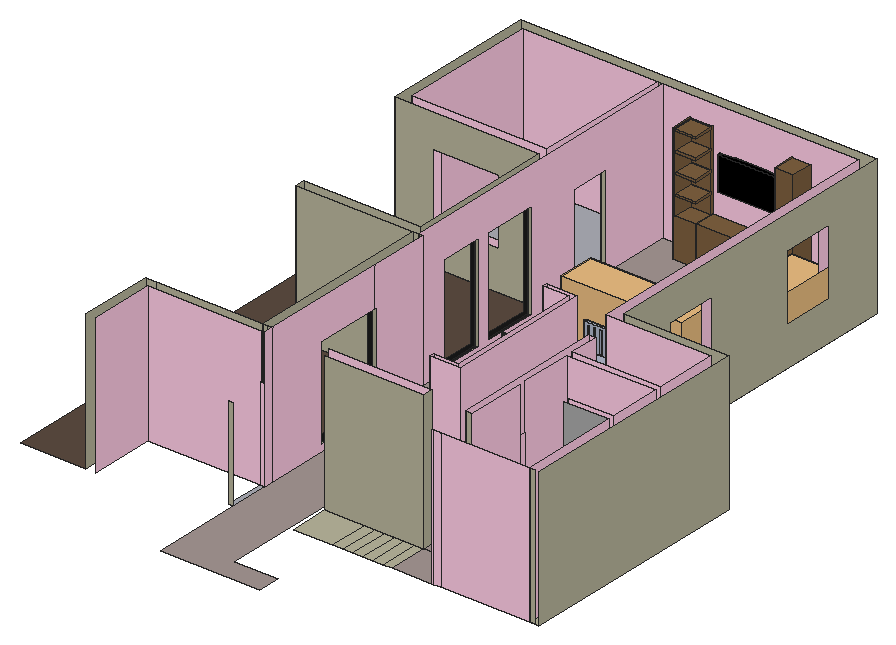
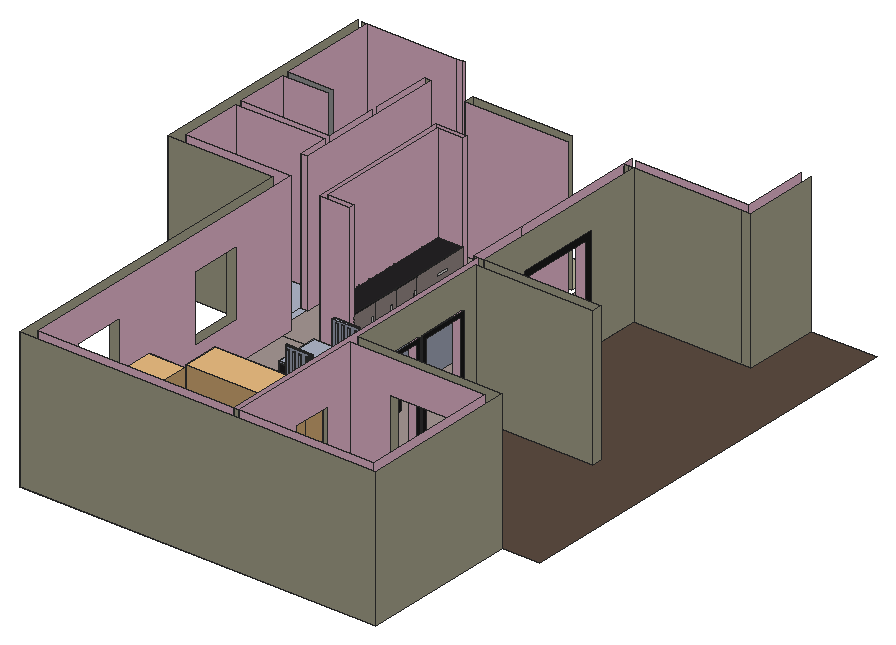
# SketchUp Ruby script. Lengths in inches.
U = 1.inch
M = Sketchup.active_model
def pt(a) = Geom::Point3d.new(a.map { |v| v * U })
def face(e, loops, mat)
  f = e.add_face(loops[0].map { |a| pt(a) })
  loops[1..].each { |l| e.add_face(l.map { |a| pt(a) }).erase! }
  f.material = f.back_material = mat if mat
  f
end
# faces: each face lists its corners as indices into pts; further lists are holes
def faces(e, pts, list, mat = nil) = list.each { |f| face(e, (f[0].is_a?(Array) ? f : [f]).map { |l| l.map { |i| pts[i] } }, mat) }
# xy, xz, yz: faces in a plane at the given z, y or x. An outline is a flat list of corners, or four numbers for a rectangle; further outlines are holes
def ring(l) = l.size == 4 ? [[l[0], l[1]], [l[2], l[1]], [l[2], l[3]], [l[0], l[3]]] : l.each_slice(2).to_a
def flat(e, list, mat, &to3) = list.each { |f| face(e, (f[0].is_a?(Array) ? f : [f]).map { |l| ring(l).map { |u, v| to3.(u, v) } }, mat) }
def xy(e, z, list, mat = nil) = flat(e, list, mat) { |x, y| [x, y, z] }
def xz(e, y, list, mat = nil) = flat(e, list, mat) { |x, z| [x, y, z] }
def yz(e, x, list, mat = nil) = flat(e, list, mat) { |y, z| [x, y, z] }
def lines(e, pts, list) = list.each { |a, b| e.add_line(pt(pts[a]), pt(pts[b])) }
# prism: a flat outline (further loops are holes) pulled along v
def prism(e, loops, v, mat = nil)
  f = face(e, loops, mat); d = Geom::Vector3d.new(v.map { |x| x * U })
  f.pushpull(f.normal.samedirection?(d) ? d.length : -d.length)
end
def box(e, o, s, mat = nil) = prism(e, [[o, [o[0] + s[0], o[1], o[2]], [o[0] + s[0], o[1] + s[1], o[2]], [o[0], o[1] + s[1], o[2]]]], [0, 0, s[2]], mat)
def at(x, y, z, deg = 0) = Geom::Transformation.translation(pt([x, y, z])) * Geom::Transformation.rotation(ORIGIN, Z_AXIS, deg.degrees)
def axes(o, x, y, z) = Geom::Transformation.new([*x, 0, *y, 0, *z, 0, *pt(o).to_a, 1])
def part(name) = M.definitions.add(name)
# library, detail: a bought-in or finely detailed component or shape, given as its bounding box
def library(name, o, s) = part(name).tap { |d| box(d.entities, o, s) }
def detail(e, o, s) = box(e.add_group.entities, o, s)
def put(e, d, t, mat = nil) = e.add_instance(d, t).tap { |i| i.material = mat if mat }
def group(e, t, mat = nil) = e.add_group.tap { |g| g.transformation = t; g.material = mat if mat }.entities
root = M.entities
M.materials.add("A01_Blush_Petal").color = [255, 204, 204]
M.materials.add("Concrete_04_1K").color = [184, 181, 156]
M.materials.add("L01_Cotton_Candy").color = [255, 204, 229]
M.materials.add("M03_Pewter_Shine").color = [168, 168, 168]
M.materials.add("M08_Obsidian_Black").color = [30, 30, 30]
M.materials.add("M09_Shadow_Night").color = [0, 0, 0]
M.materials.add("Marble_03_1K").color = [175, 182, 201]
M.materials.add("Marble_06_1K").color = [165, 150, 147]
M.materials.add("Marble_07_1K").color = [36, 34, 36]
M.materials.add("Marble_20_1K").color = [172, 173, 182]
M.materials.add("Metal_06_1K").color = [238, 236, 231]
M.materials.add("Plywood_01_1K").color = [125, 96, 64]
M.materials.add("Wood_Floor_12_1K1").color = [92, 75, 65]
c1 = part("Group\#36")
box(c1.entities,[0,0,0],[9.75,2,0.5],"Metal_06_1K")
c2 = part("Group\#37")
box(c2.entities,[0,0,0],[1.1875,6.9375,0.5],"Metal_06_1K")
c3 = part("Group\#33")
box(c3.entities,[0,0,0],[0.9375,5.25,0.5625],"Metal_06_1K")
c4 = part("Group\#34")
box(c4.entities,[0,0,0],[5.4375,1.0625,0.5625],"Metal_06_1K")
c5 = part("Group\#40")
xy(c5.entities,24,[[0,0,3,3],[21,0,24,3],[0,21,3,24],[21,21,24,24]],"Marble_07_1K")
xz(c5.entities,0,[[0,0,3,24],[21,0,24,24]],"Marble_07_1K")
xz(c5.entities,3,[[0,0,3,24],[21,0,24,24]],"Marble_07_1K")
xz(c5.entities,21,[[0,0,3,24],[21,0,24,24]],"Marble_07_1K")
xz(c5.entities,24,[[0,0,3,24],[21,0,24,24]],"Marble_07_1K")
yz(c5.entities,0,[[0,0,3,24],[21,0,24,24]],"Marble_07_1K")
yz(c5.entities,3,[[0,0,3,24],[21,0,24,24]],"Marble_07_1K")
yz(c5.entities,21,[[0,0,3,24],[21,0,24,24]],"Marble_07_1K")
yz(c5.entities,24,[[0,0,3,24],[21,0,24,24]],"Marble_07_1K")
c6 = library("Group\#54",[-38,-24.71,0],[56.29,56.29,30.0625])
c7 = part("Group\#53")
box(c7.entities,[0,0,0],[18.75,17.875,2],"Plywood_01_1K")
xy(root,15,[[4865.8125,3833.04,4865.8125,3923.04,4825.3125,3923.04,4825.3125,3929.04,4865.8125,3929.04,4865.8125,3977.04,4784.8125,3977.04,4784.8125,3869.04,4778.8125,3869.04,4778.8125,4010.04,4784.8125,4010.04,4784.8125,3983.04,4865.8125,3983.04,4865.8125,4040.04,4769.8125,4040.04,4769.8125,4328.04,4463.8125,4328.04,4463.8125,4202.04,4591.8125,4202.04,4591.8125,4049.04,4480,4049.04,4480,4058.04,4586.8125,4058.04,4586.8125,4193.04,4454.8125,4193.04,4454.8125,4337.04,4778.8125,4337.04,4778.8125,4049.04,4874.8125,4049.04,4874.8125,3833.04],[4650.8125,3833.04,4686.8125,3869.04],[4686.8125,3833.04,4696.125,3869.04],[4696.125,3833.04,4705.125,3869.04],[4705.125,3833.04,4714.125,3869.04],
  [4714.125,3833.04,4723.125,3869.04],[4723.125,3833.04,4732.125,3869.04],[4732.125,3833.04,4741.125,3869.04],[4586.8125,3878.04,4595.8125,4049.04],[4708.76,3915.92,4708.76,3919.92,4732.01,3919.92,4732.01,4045.04,4708.76,4045.04,4708.76,4049.04,4736.64,4049.04,4736.64,3915.92],
  [4586.8125,4202.04,4591.8125,4226.61],[4586.8125,4262.61,4591.8125,4328.04]],"Concrete_04_1K")
xy(root,15,[[4584.8125,4073.96,4586.8125,4121.29],[4584.8125,4124.29,4586.8125,4181.29]],"M08_Obsidian_Black")
xy(root,15,[[4778.8125,3833.04,4784.8125,3869.04],[4784.8125,3833.04,4865.8125,3833.04,4865.8125,3923.04,4825.3125,3923.04,4825.3125,3929.04,4865.8125,3929.04,4865.8125,3977.04,4784.8125,3977.04],[4784.8125,3983.04,4865.8125,4040.04],[4778.8125,4010.04,4784.8125,4040.04]],"Marble_03_1K")
xy(root,15,[[4595.8125,3750.01,4686.8125,3750.01,4686.8125,3770.04,4646.8125,3770.04,4646.8125,3878.04,4650.8125,3878.04,4650.8125,3994.42,4595.8125,3994.42],[4741.125,3833.04,4778.8125,3869.04],[4741.125,3869.04,4778.8125,3878.04],[4650.8125,3878.04,4778.8125,3878.04,4778.8125,4040.04,4769.8125,4040.04,4769.8125,4049.04,4736.64,4049.04,4736.64,3915.92,4708.76,3915.92,4708.76,4049.04,4595.8125,4049.04,4595.8125,3994.42,4650.8125,3994.42,4650.8125,4044.23,4674.8125,4044.23,4674.8125,3936.23,4650.8125,3936.23],[4591.8125,4049.04,4769.8125,4049.04,4769.8125,4328.04,4591.8125,4328.04,4591.8125,4262.61,4586.8125,4262.61,4586.8125,4226.61,4591.8125,4226.61]],"Marble_06_1K")
xy(root,15,[[4591.8125,3833.04,4595.8125,3869.04],[4463.8125,4202.04,4586.8125,4328.04]],"Marble_20_1K")
xy(root,15,[[4420.38,3809.79,4480,3809.79,4480,3878.04,4586.8125,3878.04,4586.8125,4049.04,4480,4049.04,4480,4058.04,4586.8125,4058.04,4586.8125,4073.96,4584.8125,4073.96,4584.8125,4121.29,4586.8125,4121.29,4586.8125,4124.29,4584.8125,4124.29,4584.8125,4181.29,4586.8125,4181.29,4586.8125,4193.04,4420.38,4193.04]],"Wood_Floor_12_1K1")
xz(root,3833.04,[[4591.8125,15,4595.8125,99],[4865.8125,15,4870.8125,141]],"Concrete_04_1K")
xz(root,3833.04,[[4777.125,15,4778.8125,141],[4778.8125,15,4784.8125,141],[4784.8125,15,4865.8125,141]],"L01_Cotton_Candy")
xz(root,3869.04,[[4650.8125,15,4741.125,141],[4778.8125,15,4784.8125,141]],"Concrete_04_1K")
xz(root,3869.04,[[4489,15,4591.8125,141],[4591.8125,15,4595.8125,99]],"L01_Cotton_Candy")
xz(root,3878.04,[[4480,15,4489,141],[4489,15,4586.8125,141],[4586.8125,15,4591.8125,141],[4591.8125,15,4595.8125,141]],"Concrete_04_1K")
xz(root,3878.04,[[4646.8125,15,4741.125,141]],"L01_Cotton_Candy")
xz(root,3915.92,[[4708.76,15,4736.64,141]],"L01_Cotton_Candy")
xz(root,3919.92,[[4708.76,15,4732.01,141]],"L01_Cotton_Candy")
xz(root,3923.04,[[4825.3125,15,4865.8125,141]],"M03_Pewter_Shine")
xz(root,3929.04,[[4825.3125,15,4865.8125,141]],"L01_Cotton_Candy")
xz(root,3977.04,[[4784.8125,15,4865.8125,141]],"L01_Cotton_Candy")
xz(root,3983.04,[[4784.8125,15,4865.8125,141]],"L01_Cotton_Candy")
xz(root,4010.04,[[4778.8125,15,4784.8125,141]],"L01_Cotton_Candy")
xz(root,4040.04,[[4769.8125,15,4865.8125,141]],"L01_Cotton_Candy")
xz(root,4045.04,[[4708.76,15,4732.01,141]],"L01_Cotton_Candy")
xz(root,4049.04,[[4480,15,4586.8125,141],[4586.8125,15,4591.8125,141],[4591.8125,15,4595.8125,141],[4778.8125,15,4874.8125,141]],"Concrete_04_1K")
xz(root,4049.04,[[4708.76,15,4736.64,141]],"L01_Cotton_Candy")
xz(root,4058.04,[[4480,15,4586.8125,141]],"Concrete_04_1K")
xz(root,4073.96,[[4584.8125,15,4586.8125,111]],"M08_Obsidian_Black")
xz(root,4121.29,[[4584.8125,15,4586.8125,111]],"M08_Obsidian_Black")
xz(root,4124.29,[[4584.8125,15,4586.8125,111]],"M08_Obsidian_Black")
xz(root,4181.29,[[4584.8125,15,4586.8125,111]],"M08_Obsidian_Black")
xz(root,4193.04,[[[4454.8125,15,4586.8125,141],[4489.8125,51,4549.8125,111]]],"Concrete_04_1K")
xz(root,4202.04,[[[4463.8125,15,4586.8125,141],[4489.8125,51,4549.8125,111]]],"L01_Cotton_Candy")
xz(root,4226.61,[[4586.8125,15,4591.8125,99]],"Concrete_04_1K")
xz(root,4262.61,[[4586.8125,15,4591.8125,99]],"Concrete_04_1K")
xz(root,4328.04,[[4586.8125,15,4591.8125,141]],"Concrete_04_1K")
xz(root,4328.04,[[4463.8125,15,4586.8125,141],[4591.8125,15,4769.8125,141]],"L01_Cotton_Candy")
xz(root,4337.04,[[4454.8125,15,4778.8125,141]],"Concrete_04_1K")
yz(root,4454.8125,[[4193.04,15,4337.04,141]],"Concrete_04_1K")
yz(root,4463.8125,[[4202.04,15,4328.04,141]],"L01_Cotton_Candy")
yz(root,4480,[[3809.79,15,3878.04,141],[4049.04,15,4058.04,141]],"Concrete_04_1K")
yz(root,4489,[[3809.79,15,3869.04,141]],"L01_Cotton_Candy")
yz(root,4584.8125,[[[4073.96,15,4121.29,111],[4077.51,18.55,4117.75,107.45]],[[4124.29,15,4181.29,111],[4127.84,18.55,4177.75,107.45]]],"M08_Obsidian_Black")
yz(root,4586.8125,[[3878.04,15,3878.04,141,4049.04,141,4049.04,15,4003.17,15,4003.17,111,3926.48,111,3926.48,15],[4058.04,15,4058.04,141,4193.04,141,4193.04,15,4181.29,15,4181.29,111,4124.29,111,4124.29,15,4121.29,15,4121.29,111,4073.96,111,4073.96,15]],"Concrete_04_1K")
yz(root,4586.8125,[[4202.04,15,4202.04,141,4328.04,141,4328.04,15,4262.61,15,4262.61,99,4226.61,99,4226.61,15]],"L01_Cotton_Candy")
yz(root,4586.8125,[[[3926.48,15,4003.17,111],[3932.41,20.93,3997.24,105.07]]],"M08_Obsidian_Black")
yz(root,4591.8125,[[[4049.04,15,4226.61,15,4226.61,99,4262.61,99,4262.61,15,4328.04,15,4328.04,141,4049.04,141],[4127.84,18.55,4177.75,107.45],[4077.51,18.55,4117.75,107.45]]],"L01_Cotton_Candy")
yz(root,4595.8125,[[3869.04,15,3878.04,141],[3878.04,15,3994.42,15,3994.42,20.93,3932.41,20.93,3932.41,105.07,3994.42,105.07,3994.42,141,3878.04,141],[3994.42,15,4049.04,15,4049.04,141,3994.42,141,3994.42,105.07,3997.24,105.07,3997.24,20.93,3994.42,20.93]],"L01_Cotton_Candy")
yz(root,4708.76,[[3915.92,15,3919.92,141],[4045.04,15,4049.04,141]],"L01_Cotton_Candy")
yz(root,4732.01,[[3919.92,15,4045.04,141]],"L01_Cotton_Candy")
yz(root,4736.64,[[3915.92,15,4049.04,141]],"L01_Cotton_Candy")
yz(root,4741.125,[[3869.04,15,3878.04,141]],"Concrete_04_1K")
yz(root,4769.8125,[[[4040.04,15,4328.04,141],[4101.42,51,4149.42,111],[4234.61,51,4282.61,111]]],"L01_Cotton_Candy")
yz(root,4778.8125,[[[4049.04,15,4337.04,141],[4234.61,51,4282.61,111],[4101.42,51,4149.42,111]]],"Concrete_04_1K")
yz(root,4778.8125,[[3869.04,15,4010.04,141]],"L01_Cotton_Candy")
yz(root,4784.8125,[[3869.04,15,3923.04,141],[3923.04,15,3929.04,99],[3929.04,15,3977.04,141],[3983.04,15,4010.04,141]],"L01_Cotton_Candy")
yz(root,4825.3125,[[3923.04,15,3929.04,99]],"Concrete_04_1K")
yz(root,4865.8125,[[3833.04,15,3923.04,141],[3929.04,15,3977.04,141],[3983.04,15,4040.04,141]],"L01_Cotton_Candy")
yz(root,4874.8125,[[3833.04,15,4049.04,141]],"Concrete_04_1K")
g1 = group(root,at(4708.76,3919.92,15))
xy(g1,0,[[0,0,23.25,125.125]],"Marble_06_1K")
xy(g1,36,[[0,0,23.25,125.125]],"Marble_07_1K")
xy(g1,37,[[0,0,23.25,125.125]],"Marble_07_1K")
xz(g1,0,[[0,0,23.25,36]],"Marble_06_1K")
xz(g1,0,[[0,36,23.25,37]],"Marble_07_1K")
xz(g1,125.125,[[0,0,23.25,36]],"Marble_06_1K")
xz(g1,125.125,[[0,36,23.25,37]],"Marble_07_1K")
yz(g1,0,[[0,0,53.125,18],[53.125,0,77.125,36],[77.125,0,101.125,36],[101.125,0,125.125,36],[0,18,53.125,36]],"Marble_06_1K")
yz(g1,0,[[0,36,77.125,37],[77.125,36,125.125,37]],"Marble_07_1K")
yz(g1,23.25,[[0,0,125.125,36]],"Marble_06_1K")
yz(g1,23.25,[[0,36,125.125,37]],"Marble_07_1K")
put(g1,c1,axes([0,29.32,26.15],[0,-1,0],[0,0,1],[-1,0,0]),"Metal_06_1K")
put(g1,c1,axes([0,31.12,11.2],[0,-1,0],[0,0,1],[-1,0,0]),"Metal_06_1K")
put(g1,c2,axes([0,56.34,18.51],[0,-1,0],[0,0,1],[-1,0,0]))
put(g1,c2,axes([0,83.09,18.51],[0,-1,0],[0,0,1],[-1,0,0]))
put(g1,c2,axes([0,105.28,18.51],[0,-1,0],[0,0,1],[-1,0,0]))
g2 = group(root,at(4650.8125,3936.23,15))
xy(g2,0,[[0,0,24,108]],"Marble_03_1K")
xy(g2,36,[[0,0,24,108]],"Marble_07_1K")
xy(g2,37,[[0,0,24,108]],"Marble_07_1K")
xz(g2,0,[[0,0,24,36]],"Marble_03_1K")
xz(g2,0,[[0,36,24,37]],"Marble_07_1K")
xz(g2,108,[[0,0,24,36]],"Marble_03_1K")
xz(g2,108,[[0,36,24,37]],"Marble_07_1K")
yz(g2,0,[[0,0,108,36]],"Marble_03_1K")
yz(g2,0,[[0,36,58.1875,37],[58.1875,36,108,37]],"Marble_07_1K")
yz(g2,24,[[0,0,24,36],[24,0,48,36],[48,0,84,9],[84,0,108,36],[48,9,84,18],
  [48,18,84,27],[48,27,84,36]],"Marble_03_1K")
yz(g2,24,[[0,36,108,37]],"Marble_07_1K")
put(g2,c3,axes([24,85.05,22.03],[0,1,0],[0,0,1],[1,0,0]),"Metal_06_1K")
put(g2,c3,axes([24,45.67,22.03],[0,1,0],[0,0,1],[1,0,0]),"Metal_06_1K")
put(g2,c3,axes([24,22.05,22.03],[0,1,0],[0,0,1],[1,0,0]),"Metal_06_1K")
put(g2,c4,axes([24,64.03,31.23],[0,1,0],[0,0,1],[1,0,0]))
put(g2,c4,axes([24,64.03,22.79],[0,1,0],[0,0,1],[1,0,0]))
put(g2,c4,axes([24,64.03,11.85],[0,1,0],[0,0,1],[1,0,0]))
put(g2,c4,axes([24,64.03,3.04],[0,1,0],[0,0,1],[1,0,0]))
g3 = group(root,at(4668.26,4100.77,15,180))
g4 = group(g3,at(0,0,24),"Marble_03_1K")
xy(g4,0,[[0,0,0,21.71,0.1,21.95,0.22,22.19,0.35,22.43,0.5,22.65,0.66,22.86,0.84,23.07,1.03,23.26,1.23,23.43,1.4375,23.6,1.66,23.75,1.89,23.88,2.13,24,22.03,24,22.3125,23.98,22.59,23.92,22.86,23.82,23.11,23.68,23.34,23.51,23.54,23.31,23.71,23.08,23.85,22.82,23.94,22.56,24,22.29,24,0]])
xy(g4,2,[[0,0,24,21.71]])
xy(g4,3.91,[[3.32,21.71,4.94,24],[8.94,21.71,10.57,24],[14.57,21.71,16.19,24],[20.19,21.71,21.82,24]])
xy(g4,24.84,[[3.32,21.71,4.94,24],[8.94,21.71,10.57,24],[14.57,21.71,16.19,24],[20.19,21.71,21.82,24]])
xy(g4,27.0625,[[0,21.71,24,21.71,24,22.29,23.94,22.56,23.85,22.82,23.71,23.08,23.54,23.31,23.34,23.51,23.11,23.68,22.86,23.82,22.59,23.92,22.3125,23.98,22.03,24,2.13,24,1.89,23.88,1.66,23.75,1.4375,23.6,1.23,23.43,1.03,23.26,0.84,23.07,0.66,22.86,0.5,22.65,0.35,22.43,0.22,22.19,0.1,21.95],[24,21.71,24.02,21.99,24,22.28,24,22.29]])
xz(g4,0,[[0,0,24,2]])
xz(g4,21.71,[[[0,2,24,27.0625],[20.19,3.91,21.82,24.84],[14.57,3.91,16.19,24.84],[8.94,3.91,10.57,24.84],[3.32,3.91,4.94,24.84]]])
xz(g4,24,[[[2.13,0,22.03,27.0625],[20.19,3.91,21.82,24.84],[14.57,3.91,16.19,24.84],[8.94,3.91,10.57,24.84],[3.32,3.91,4.94,24.84]]])
yz(g4,0,[[0,0,21.71,2]])
yz(g4,3.32,[[21.71,3.91,24,24.84]])
yz(g4,4.94,[[21.71,3.91,24,24.84]])
yz(g4,8.94,[[21.71,3.91,24,24.84]])
yz(g4,10.57,[[21.71,3.91,24,24.84]])
yz(g4,14.57,[[21.71,3.91,24,24.84]])
yz(g4,16.19,[[21.71,3.91,24,24.84]])
yz(g4,20.19,[[21.71,3.91,24,24.84]])
yz(g4,21.82,[[21.71,3.91,24,24.84]])
yz(g4,24,[[0,0,22.29,0,22.29,27.0625,21.71,27.0625,21.71,2,0,2]])
p = [[0,21.71,27.0625],[0.1,21.95,27.0625],[0.1,21.95,0],[0,21.71,0],[0,21.71,2],[0.22,22.19,27.0625],
  [0.22,22.19,0],[0.35,22.43,27.0625],[0.35,22.43,0],[23.94,22.56,27.0625],[24,22.29,27.0625],[24,22.29,0],
  [23.94,22.56,0],[0.5,22.65,27.0625],[0.5,22.65,0],[23.85,22.82,27.0625],[23.85,22.82,0],[0.66,22.86,27.0625],
  [0.66,22.86,0],[23.71,23.08,27.0625],[23.71,23.08,0],[0.84,23.07,27.0625],[0.84,23.07,0],[1.03,23.26,27.0625],
  [1.03,23.26,0],[23.54,23.31,27.0625],[23.54,23.31,0],[1.23,23.43,27.0625],[1.23,23.43,0],[23.34,23.51,27.0625],
  [23.34,23.51,0],[1.4375,23.6,27.0625],[1.4375,23.6,0],[23.11,23.68,27.0625],[23.11,23.68,0],[1.66,23.75,27.0625],
  [1.66,23.75,0],[1.89,23.88,27.0625],[1.89,23.88,0],[22.86,23.82,27.0625],[22.86,23.82,0],[22.59,23.92,27.0625],
  [22.59,23.92,0],[2.13,24,27.0625],[2.13,24,0],[22.3125,23.98,27.0625],[22.3125,23.98,0],[22.03,24,27.0625],
  [22.03,24,0]]
faces(g4,p,[[0,1,2,3,4],[1,5,6,2],[5,7,8,6],[9,10,11,12],[7,13,14,8],[15,9,12,16],[13,17,18,14],[19,15,16,20],
  [17,21,22,18],[21,23,24,22],[25,19,20,26],[23,27,28,24],[29,25,26,30],[27,31,32,28],[33,29,30,34],[31,35,36,32],
  [35,37,38,36],[39,33,34,40],[41,39,40,42],[37,43,44,38],[45,41,42,46],[47,45,46,48]])
put(g3,c5,at(0,0,0))
g5 = group(root,at(4700.88,4100.77,15,180))
g6 = group(g5,at(0,0,24),"Marble_03_1K")
xy(g6,0,[[0,0,0,21.705,0.033,21.948,0.087,22.187,0.162,22.42,0.257,22.646,0.371,22.863,0.503,23.069,0.653,23.263,0.819,23.443,1,23.608,1.195,23.756,1.402,23.887,1.62,24,22.38,24,22.619,23.918,22.848,23.81,23.063,23.676,23.261,23.518,23.441,23.339,23.598,23.141,23.732,22.926,23.841,22.697,23.923,22.458,23.977,22.21,24,21.989,24,0]])
xy(g6,2,[[0,0,24,21.705]])
xy(g6,3.906,[[3.317,21.705,4.942,24],[8.942,21.705,10.567,24],[14.567,21.705,16.192,24],[20.192,21.705,21.817,24]])
xy(g6,24.844,[[3.317,21.705,4.942,24],[8.942,21.705,10.567,24],[14.567,21.705,16.192,24],[20.192,21.705,21.817,24]])
xy(g6,27.0625,[[0,21.705,24,21.705,24,21.989,23.977,22.21,23.923,22.458,23.841,22.697,23.732,22.926,23.598,23.141,23.441,23.339,23.261,23.518,23.063,23.676,22.848,23.81,22.619,23.918,22.38,24,1.62,24,1.402,23.887,1.195,23.756,1,23.608,0.819,23.443,0.653,23.263,0.503,23.069,0.371,22.863,0.257,22.646,0.162,22.42,0.087,22.187,0.033,21.948],[24,21.705,24.003,21.958,24,21.989]])
xz(g6,0,[[0,0,24,2]])
xz(g6,21.705,[[[0,2,24,27.0625],[20.192,3.906,21.817,24.844],[14.567,3.906,16.192,24.844],[8.942,3.906,10.567,24.844],[3.317,3.906,4.942,24.844]]])
xz(g6,24,[[[1.62,0,22.38,27.0625],[20.192,3.906,21.817,24.844],[14.567,3.906,16.192,24.844],[8.942,3.906,10.567,24.844],[3.317,3.906,4.942,24.844]]])
yz(g6,0,[[0,0,21.705,2]])
yz(g6,3.317,[[21.705,3.906,24,24.844]])
yz(g6,4.942,[[21.705,3.906,24,24.844]])
yz(g6,8.942,[[21.705,3.906,24,24.844]])
yz(g6,10.567,[[21.705,3.906,24,24.844]])
yz(g6,14.567,[[21.705,3.906,24,24.844]])
yz(g6,16.192,[[21.705,3.906,24,24.844]])
yz(g6,20.192,[[21.705,3.906,24,24.844]])
yz(g6,21.817,[[21.705,3.906,24,24.844]])
yz(g6,24,[[0,0,21.989,0,21.989,27.0625,21.705,27.0625,21.705,2,0,2]])
p = [[0,21.705,27.0625],[0.033,21.948,27.0625],[0.033,21.948,0],[0,21.705,0],[0,21.705,2],[0.087,22.187,27.0625],
  [0.087,22.187,0],[23.977,22.21,27.0625],[24,21.989,27.0625],[24,21.989,0],[23.977,22.21,0],[0.162,22.42,27.0625],
  [0.162,22.42,0],[23.923,22.458,27.0625],[23.923,22.458,0],[0.257,22.646,27.0625],[0.257,22.646,0],[23.841,22.697,27.0625],
  [23.841,22.697,0],[0.371,22.863,27.0625],[0.371,22.863,0],[23.732,22.926,27.0625],[23.732,22.926,0],[0.503,23.069,27.0625],
  [0.503,23.069,0],[23.598,23.141,27.0625],[23.598,23.141,0],[0.653,23.263,27.0625],[0.653,23.263,0],[23.441,23.339,27.0625],
  [23.441,23.339,0],[0.819,23.443,27.0625],[0.819,23.443,0],[23.261,23.518,27.0625],[23.261,23.518,0],[1,23.608,27.0625],
  [1,23.608,0],[23.063,23.676,27.0625],[23.063,23.676,0],[1.195,23.756,27.0625],[1.195,23.756,0],[22.848,23.81,27.0625],
  [22.848,23.81,0],[1.402,23.887,27.0625],[1.402,23.887,0],[22.619,23.918,27.0625],[22.619,23.918,0],[1.62,24,27.0625],
  [1.62,24,0],[22.38,24,27.0625],[22.38,24,0]]
faces(g6,p,[[0,1,2,3,4],[1,5,6,2],[7,8,9,10],[5,11,12,6],[13,7,10,14],[11,15,16,12],[17,13,14,18],[15,19,20,16],
  [21,17,18,22],[19,23,24,20],[25,21,22,26],[23,27,28,24],[29,25,26,30],[27,31,32,28],[33,29,30,34],[31,35,36,32],
  [37,33,34,38],[35,39,40,36],[41,37,38,42],[39,43,44,40],[45,41,42,46],[43,47,48,44],[49,45,46,50]])
put(g5,c5,at(0,0,0))
g7 = group(root,at(4635.68,4082.66,15))
xy(g7,30,[[0,0,6,6],[72.75,0,78.75,6],[0,34.375,6,40.375],[72.75,34.375,78.75,40.375]],"Marble_07_1K")
xz(g7,0,[[0,0,6,30],[72.75,0,78.75,30]],"Marble_07_1K")
xz(g7,6,[[0,0,6,30],[72.75,0,78.75,30]],"Marble_07_1K")
xz(g7,34.375,[[0,0,6,30],[72.75,0,78.75,30]],"Marble_07_1K")
xz(g7,40.375,[[0,0,6,30],[72.75,0,78.75,30]],"Marble_07_1K")
yz(g7,0,[[0,0,6,30],[34.375,0,40.375,30]],"Marble_07_1K")
yz(g7,6,[[0,0,6,30],[34.375,0,40.375,30]],"Marble_07_1K")
yz(g7,72.75,[[0,0,6,30],[34.375,0,40.375,30]],"Marble_07_1K")
yz(g7,78.75,[[0,0,6,30],[34.375,0,40.375,30]],"Marble_07_1K")
g8 = group(g7,at(0,0,30))
prism(g8,[[[0,6,0],[0,40.375,0],[6,40.375,0],[78.75,40.375,0],[78.75,34.375,0],[78.75,0,0],[72.75,0,0],[0,0,0]]],[0,0,1.4375],"Marble_03_1K")
g9 = group(root,at(4679.27,4106.38,15))
g10 = group(g9,at(0,0,24),"Marble_03_1K")
xy(g10,0,[[0,0,0,21.71,0.05,21.95,0.11,22.19,0.2,22.43,0.3,22.66,0.43,22.875,0.57,23.08,0.73,23.27,0.91,23.45,1.1,23.61,1.3,23.76,1.51,23.89,1.74,24,21.99,24,22.26,23.94,22.52,23.86,22.77,23.74,23.01,23.59,23.22,23.42,23.42,23.22,23.59,23.01,23.73,22.77,23.84,22.52,23.93,22.25,23.98,21.98,24,21.71,24,0]])
xy(g10,2,[[0,0,24,21.71]])
xy(g10,3.91,[[3.32,21.71,4.94,24],[8.94,21.71,10.57,24],[14.57,21.71,16.19,24],[20.19,21.71,21.82,24]])
xy(g10,24.84,[[3.32,21.71,4.94,24],[8.94,21.71,10.57,24],[14.57,21.71,16.19,24],[20.19,21.71,21.82,24]])
xy(g10,27.0625,[[0,21.71,24,21.71,23.98,21.98,23.93,22.25,23.84,22.52,23.73,22.77,23.59,23.01,23.42,23.22,23.22,23.42,23.01,23.59,22.77,23.74,22.52,23.86,22.26,23.94,21.99,24,1.74,24,1.51,23.89,1.3,23.76,1.1,23.61,0.91,23.45,0.73,23.27,0.57,23.08,0.43,22.875,0.3,22.66,0.2,22.43,0.11,22.19,0.05,21.95]])
xz(g10,0,[[0,0,24,2]])
xz(g10,21.71,[[[0,2,24,27.0625],[20.19,3.91,21.82,24.84],[14.57,3.91,16.19,24.84],[8.94,3.91,10.57,24.84],[3.32,3.91,4.94,24.84]]])
xz(g10,24,[[[1.74,0,21.99,27.0625],[20.19,3.91,21.82,24.84],[14.57,3.91,16.19,24.84],[8.94,3.91,10.57,24.84],[3.32,3.91,4.94,24.84]]])
yz(g10,0,[[0,0,21.71,2]])
yz(g10,3.32,[[21.71,3.91,24,24.84]])
yz(g10,4.94,[[21.71,3.91,24,24.84]])
yz(g10,8.94,[[21.71,3.91,24,24.84]])
yz(g10,10.57,[[21.71,3.91,24,24.84]])
yz(g10,14.57,[[21.71,3.91,24,24.84]])
yz(g10,16.19,[[21.71,3.91,24,24.84]])
yz(g10,20.19,[[21.71,3.91,24,24.84]])
yz(g10,21.82,[[21.71,3.91,24,24.84]])
yz(g10,24,[[0,0,21.71,2]])
p = [[0,21.71,27.0625],[0.05,21.95,27.0625],[0.05,21.95,0],[0,21.71,0],[0,21.71,2],[23.98,21.98,27.0625],
  [24,21.71,27.0625],[24,21.71,2],[24,21.71,0],[23.98,21.98,0],[0.11,22.19,27.0625],[0.11,22.19,0],
  [23.93,22.25,27.0625],[23.93,22.25,0],[0.2,22.43,27.0625],[0.2,22.43,0],[23.84,22.52,27.0625],[23.84,22.52,0],
  [0.3,22.66,27.0625],[0.3,22.66,0],[23.73,22.77,27.0625],[23.73,22.77,0],[0.43,22.875,27.0625],[0.43,22.875,0],
  [23.59,23.01,27.0625],[23.59,23.01,0],[0.57,23.08,27.0625],[0.57,23.08,0],[23.42,23.22,27.0625],[23.42,23.22,0],
  [0.73,23.27,27.0625],[0.73,23.27,0],[23.22,23.42,27.0625],[23.22,23.42,0],[0.91,23.45,27.0625],[0.91,23.45,0],
  [23.01,23.59,27.0625],[23.01,23.59,0],[1.1,23.61,27.0625],[1.1,23.61,0],[1.3,23.76,27.0625],[1.3,23.76,0],
  [22.77,23.74,27.0625],[22.77,23.74,0],[22.52,23.86,27.0625],[22.52,23.86,0],[1.51,23.89,27.0625],[1.51,23.89,0],
  [1.74,24,27.0625],[1.74,24,0],[21.99,24,27.0625],[22.26,23.94,27.0625],[22.26,23.94,0],[21.99,24,0]]
faces(g10,p,[[0,1,2,3,4],[5,6,7,8,9],[1,10,11,2],[12,5,9,13],[10,14,15,11],[16,12,13,17],[14,18,19,15],[20,16,17,21],
  [18,22,23,19],[24,20,21,25],[22,26,27,23],[28,24,25,29],[26,30,31,27],[32,28,29,33],[30,34,35,31],[36,32,33,37],
  [34,38,39,35],[38,40,41,39],[42,36,37,43],[44,42,43,45],[40,46,47,41],[46,48,49,47],[50,51,52,53],[51,44,45,52]])
put(g9,c5,at(0,0,0))
g11 = group(root,at(4646.09,4107.01,15))
g12 = group(g11,at(0,0,24),"Marble_03_1K")
xy(g12,0,[[0,0,0,21.71,0.05,21.95,0.12,22.2,0.21,22.43,0.32,22.66,0.44,22.875,0.59,23.08,0.75,23.27,0.93,23.45,1.12,23.62,1.33,23.76,1.54,23.89,1.77,24,22.13,24,22.38,23.92,22.63,23.82,22.86,23.69,23.08,23.54,23.27,23.36,23.45,23.17,23.61,22.95,23.74,22.72,23.85,22.48,23.93,22.23,23.98,21.97,24,21.71,24,0]])
xy(g12,2,[[0,0,24,21.71]])
xy(g12,3.91,[[3.32,21.71,4.94,24],[8.94,21.71,10.57,24],[14.57,21.71,16.19,24],[20.19,21.71,21.82,24]])
xy(g12,24.84,[[3.32,21.71,4.94,24],[8.94,21.71,10.57,24],[14.57,21.71,16.19,24],[20.19,21.71,21.82,24]])
xy(g12,27.0625,[[0,21.71,24,21.71,23.98,21.97,23.93,22.23,23.85,22.48,23.74,22.72,23.61,22.95,23.45,23.17,23.27,23.36,23.08,23.54,22.86,23.69,22.63,23.82,22.38,23.92,22.13,24,1.77,24,1.54,23.89,1.33,23.76,1.12,23.62,0.93,23.45,0.75,23.27,0.59,23.08,0.44,22.875,0.32,22.66,0.21,22.43,0.12,22.2,0.05,21.95]])
xz(g12,0,[[0,0,24,2]])
xz(g12,21.71,[[[0,2,24,27.0625],[20.19,3.91,21.82,24.84],[14.57,3.91,16.19,24.84],[8.94,3.91,10.57,24.84],[3.32,3.91,4.94,24.84]]])
xz(g12,24,[[[1.77,0,22.13,27.0625],[20.19,3.91,21.82,24.84],[14.57,3.91,16.19,24.84],[8.94,3.91,10.57,24.84],[3.32,3.91,4.94,24.84]]])
yz(g12,0,[[0,0,21.71,2]])
yz(g12,3.32,[[21.71,3.91,24,24.84]])
yz(g12,4.94,[[21.71,3.91,24,24.84]])
yz(g12,8.94,[[21.71,3.91,24,24.84]])
yz(g12,10.57,[[21.71,3.91,24,24.84]])
yz(g12,14.57,[[21.71,3.91,24,24.84]])
yz(g12,16.19,[[21.71,3.91,24,24.84]])
yz(g12,20.19,[[21.71,3.91,24,24.84]])
yz(g12,21.82,[[21.71,3.91,24,24.84]])
yz(g12,24,[[0,0,21.71,2]])
p = [[0,21.71,27.0625],[0.05,21.95,27.0625],[0.05,21.95,0],[0,21.71,0],[0,21.71,2],[23.98,21.97,27.0625],
  [24,21.71,27.0625],[24,21.71,2],[24,21.71,0],[23.98,21.97,0],[0.12,22.2,27.0625],[0.12,22.2,0],
  [23.93,22.23,27.0625],[23.93,22.23,0],[0.21,22.43,27.0625],[0.21,22.43,0],[23.85,22.48,27.0625],[23.85,22.48,0],
  [0.32,22.66,27.0625],[0.32,22.66,0],[23.74,22.72,27.0625],[23.74,22.72,0],[0.44,22.875,27.0625],[0.44,22.875,0],
  [23.61,22.95,27.0625],[23.61,22.95,0],[0.59,23.08,27.0625],[0.59,23.08,0],[23.45,23.17,27.0625],[23.45,23.17,0],
  [0.75,23.27,27.0625],[0.75,23.27,0],[23.27,23.36,27.0625],[23.27,23.36,0],[0.93,23.45,27.0625],[0.93,23.45,0],
  [23.08,23.54,27.0625],[23.08,23.54,0],[1.12,23.62,27.0625],[1.12,23.62,0],[22.86,23.69,27.0625],[22.86,23.69,0],
  [1.33,23.76,27.0625],[1.33,23.76,0],[22.63,23.82,27.0625],[22.63,23.82,0],[1.54,23.89,27.0625],[1.54,23.89,0],
  [22.38,23.92,27.0625],[22.38,23.92,0],[1.77,24,27.0625],[1.77,24,0],[22.13,24,27.0625],[22.13,24,0]]
faces(g12,p,[[0,1,2,3,4],[5,6,7,8,9],[1,10,11,2],[12,5,9,13],[10,14,15,11],[16,12,13,17],[14,18,19,15],[20,16,17,21],
  [18,22,23,19],[24,20,21,25],[22,26,27,23],[28,24,25,29],[26,30,31,27],[32,28,29,33],[30,34,35,31],[36,32,33,37],
  [34,38,39,35],[40,36,37,41],[38,42,43,39],[44,40,41,45],[42,46,47,43],[48,44,45,49],[46,50,51,47],[52,48,49,53]])
put(g11,c5,at(0,0,0))
g13 = group(root,at(4632.15,4168.6,15),"A01_Blush_Petal")
detail(g13,[-3.4375,-3,0],[109.625,33.5,53.0625])
g14 = group(root,at(4766.8125,4205.22,15),"A01_Blush_Petal")
detail(g14,[-30.5,-2.85,0],[33.5,90.99,53.0625])
put(root,c6,at(4702.42,4249,15))
g15 = group(root,at(4637.1875,4308.17,15))
prism(g15,[[[30.25,19.81,58.32],[34.75,19.875,58.32],[39.25,19.81,58.32],[43.74,19.63,58.32],[48.23,19.34,58.32],[52.71,18.92,58.32],[57.17,18.375,58.32],[61.625,17.72,58.32],[61.625,15.5625,58.32],[7.875,15.5625,58.32],[7.875,17.72,58.32],[12.32,18.375,58.32],[16.79,18.92,58.32],[21.27,19.34,58.32],[25.76,19.63,58.32]]],[0,0,30.4375],"M09_Shadow_Night")
xy(g15,0,[[-20.75,0,0,19.875],[0,0,72.1875,19.875],[72.1875,0,89,19.875]],"Plywood_01_1K")
xy(g15,36,[[0,0,72.1875,19.875]],"Plywood_01_1K")
xy(g15,107.1875,[[-20.75,0,-18.75,0,-18.75,17.875,0,17.875,0,19.875,-20.75,19.875],[72.1875,0,89,19.875]],"Plywood_01_1K")
xz(g15,0,[[-20.75,0,0,0,0,36,-18.75,36,-18.75,107.1875,-20.75,107.1875],[0,0,72.1875,36],[72.1875,0,89,107.1875]],"Plywood_01_1K")
xz(g15,17.875,[[-18.75,36,0,107.1875]],"Plywood_01_1K")
xz(g15,19.875,[[-20.75,0,0,107.1875],[0,0,72.1875,36],[72.1875,0,89,107.1875]],"Plywood_01_1K")
yz(g15,-20.75,[[0,0,19.875,107.1875]],"Plywood_01_1K")
yz(g15,-18.75,[[0,36,17.875,107.1875]],"Plywood_01_1K")
yz(g15,0,[[0,0,19.875,36],[17.875,36,19.875,107.1875]],"Plywood_01_1K")
yz(g15,72.1875,[[0,0,19.875,36],[0,36,19.875,107.1875]],"Plywood_01_1K")
yz(g15,89,[[0,0,19.875,107.1875]],"Plywood_01_1K")
g16 = group(g15,at(-18.75,0,36))
xy(g16,0,[[0,0,18.75,17.875]],"Plywood_01_1K")
put(g15,c7,at(-18.75,0,52.3125))
put(g15,c7,at(-18.75,0,70.02))
put(g15,c7,at(-18.75,0,87.73))
g17 = group(g15,at(-18.75,0,105.4375))
box(g17,[0,0,0],[18.75,17.875,2],"Plywood_01_1K")
